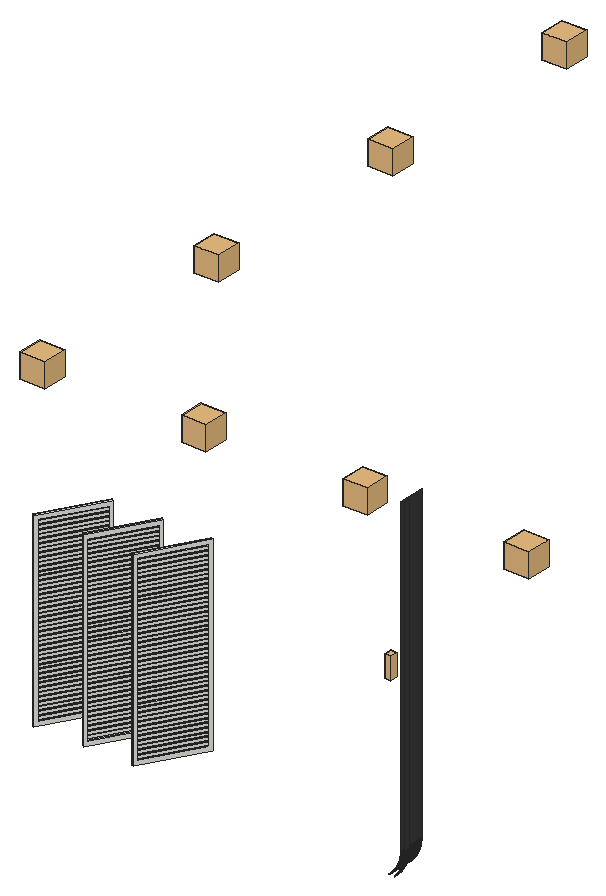
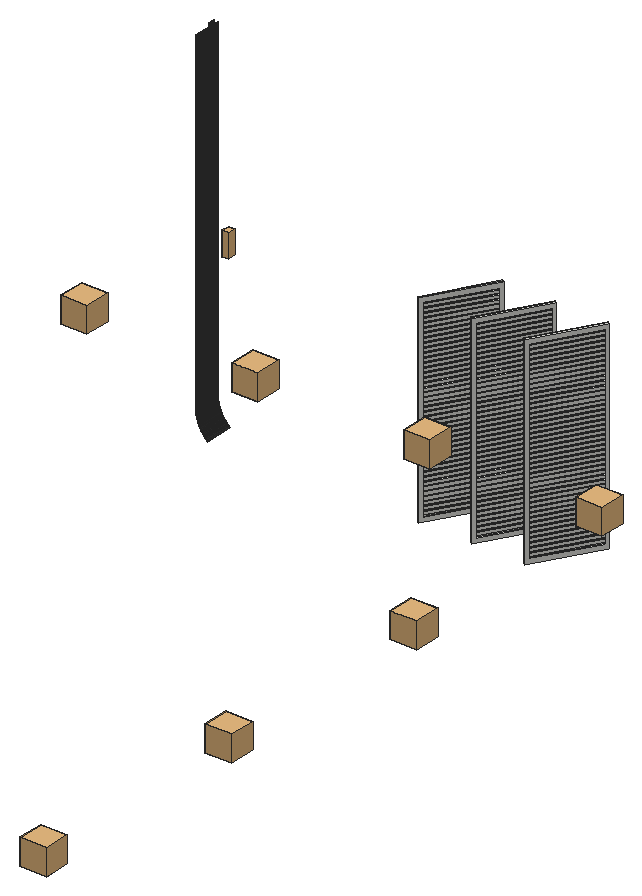
# SketchUp Ruby script. Lengths in inches.
U = 1.inch
M = Sketchup.active_model
def pt(a) = Geom::Point3d.new(a.map { |v| v * U })
def face(e, loops, mat)
  f = e.add_face(loops[0].map { |a| pt(a) })
  loops[1..].each { |l| e.add_face(l.map { |a| pt(a) }).erase! }
  f.material = f.back_material = mat if mat
  f
end
# faces: each face lists its corners as indices into pts; further lists are holes
def faces(e, pts, list, mat = nil) = list.each { |f| face(e, (f[0].is_a?(Array) ? f : [f]).map { |l| l.map { |i| pts[i] } }, mat) }
# xy, xz, yz: faces in a plane at the given z, y or x. An outline is a flat list of corners, or four numbers for a rectangle; further outlines are holes
def ring(l) = l.size == 4 ? [[l[0], l[1]], [l[2], l[1]], [l[2], l[3]], [l[0], l[3]]] : l.each_slice(2).to_a
def flat(e, list, mat, &to3) = list.each { |f| face(e, (f[0].is_a?(Array) ? f : [f]).map { |l| ring(l).map { |u, v| to3.(u, v) } }, mat) }
def xy(e, z, list, mat = nil) = flat(e, list, mat) { |x, y| [x, y, z] }
def xz(e, y, list, mat = nil) = flat(e, list, mat) { |x, z| [x, y, z] }
def yz(e, x, list, mat = nil) = flat(e, list, mat) { |y, z| [x, y, z] }
def lines(e, pts, list) = list.each { |a, b| e.add_line(pt(pts[a]), pt(pts[b])) }
# prism: a flat outline (further loops are holes) pulled along v
def prism(e, loops, v, mat = nil)
  f = face(e, loops, mat); d = Geom::Vector3d.new(v.map { |x| x * U })
  f.pushpull(f.normal.samedirection?(d) ? d.length : -d.length)
end
def box(e, o, s, mat = nil) = prism(e, [[o, [o[0] + s[0], o[1], o[2]], [o[0] + s[0], o[1] + s[1], o[2]], [o[0], o[1] + s[1], o[2]]]], [0, 0, s[2]], mat)
def at(x, y, z, deg = 0) = Geom::Transformation.translation(pt([x, y, z])) * Geom::Transformation.rotation(ORIGIN, Z_AXIS, deg.degrees)
def axes(o, x, y, z) = Geom::Transformation.new([*x, 0, *y, 0, *z, 0, *pt(o).to_a, 1])
def part(name) = M.definitions.add(name)
# library, detail: a bought-in or finely detailed component or shape, given as its bounding box
def library(name, o, s) = part(name).tap { |d| box(d.entities, o, s) }
def detail(e, o, s) = box(e.add_group.entities, o, s)
def put(e, d, t, mat = nil) = e.add_instance(d, t).tap { |i| i.material = mat if mat }
def group(e, t, mat = nil) = e.add_group.tap { |g| g.transformation = t; g.material = mat if mat }.entities
root = M.entities
M.materials.add("1496 AP 8293 CARBON COPY").color = [58, 58, 58]
c1 = part("1")
box(c1.entities,[-0.25,-0.25,0],[1,1,33])
c2 = part("Group\#27")
prism(c2.entities,[[[36,0,0],[0,0,0],[0,0,72],[36,0,72]],[[34.5,0,1.5],[34.5,0,70.5],[1.5,0,70.5],[1.5,0,1.5]]],[0,-1.5,0])
put(c2.entities,c1,axes([1.5,-1,2.5],[0,1,0],[0,0,1],[1,0,0]))
put(c2.entities,c1,axes([1.5,-1,4.08],[0,1,0],[0,0,1],[1,0,0]))
put(c2.entities,c1,axes([1.5,-1,5.67],[0,1,0],[0,0,1],[1,0,0]))
put(c2.entities,c1,axes([1.5,-1,7.25],[0,1,0],[0,0,1],[1,0,0]))
put(c2.entities,c1,axes([1.5,-1,8.83],[0,1,0],[0,0,1],[1,0,0]))
put(c2.entities,c1,axes([1.5,-1,10.42],[0,1,0],[0,0,1],[1,0,0]))
put(c2.entities,c1,axes([1.5,-1,12],[0,1,0],[0,0,1],[1,0,0]))
put(c2.entities,c1,axes([1.5,-1,13.58],[0,1,0],[0,0,1],[1,0,0]))
put(c2.entities,c1,axes([1.5,-1,15.17],[0,1,0],[0,0,1],[1,0,0]))
put(c2.entities,c1,axes([1.5,-1,16.75],[0,1,0],[0,0,1],[1,0,0]))
put(c2.entities,c1,axes([1.5,-1,18.33],[0,1,0],[0,0,1],[1,0,0]))
put(c2.entities,c1,axes([1.5,-1,19.92],[0,1,0],[0,0,1],[1,0,0]))
put(c2.entities,c1,axes([1.5,-1,21.5],[0,1,0],[0,0,1],[1,0,0]))
put(c2.entities,c1,axes([1.5,-1,23.08],[0,1,0],[0,0,1],[1,0,0]))
put(c2.entities,c1,axes([1.5,-1,24.67],[0,1,0],[0,0,1],[1,0,0]))
put(c2.entities,c1,axes([1.5,-1,26.25],[0,1,0],[0,0,1],[1,0,0]))
put(c2.entities,c1,axes([1.5,-1,27.83],[0,1,0],[0,0,1],[1,0,0]))
put(c2.entities,c1,axes([1.5,-1,29.42],[0,1,0],[0,0,1],[1,0,0]))
put(c2.entities,c1,axes([1.5,-1,31],[0,1,0],[0,0,1],[1,0,0]))
put(c2.entities,c1,axes([1.5,-1,32.58],[0,1,0],[0,0,1],[1,0,0]))
put(c2.entities,c1,axes([1.5,-1,34.17],[0,1,0],[0,0,1],[1,0,0]))
put(c2.entities,c1,axes([1.5,-1,35.75],[0,1,0],[0,0,1],[1,0,0]))
put(c2.entities,c1,axes([1.5,-1,37.33],[0,1,0],[0,0,1],[1,0,0]))
put(c2.entities,c1,axes([1.5,-1,38.92],[0,1,0],[0,0,1],[1,0,0]))
put(c2.entities,c1,axes([1.5,-1,40.5],[0,1,0],[0,0,1],[1,0,0]))
put(c2.entities,c1,axes([1.5,-1,42.08],[0,1,0],[0,0,1],[1,0,0]))
put(c2.entities,c1,axes([1.5,-1,43.67],[0,1,0],[0,0,1],[1,0,0]))
put(c2.entities,c1,axes([1.5,-1,45.25],[0,1,0],[0,0,1],[1,0,0]))
put(c2.entities,c1,axes([1.5,-1,46.83],[0,1,0],[0,0,1],[1,0,0]))
put(c2.entities,c1,axes([1.5,-1,48.42],[0,1,0],[0,0,1],[1,0,0]))
put(c2.entities,c1,axes([1.5,-1,50],[0,1,0],[0,0,1],[1,0,0]))
put(c2.entities,c1,axes([1.5,-1,51.58],[0,1,0],[0,0,1],[1,0,0]))
put(c2.entities,c1,axes([1.5,-1,53.17],[0,1,0],[0,0,1],[1,0,0]))
put(c2.entities,c1,axes([1.5,-1,54.75],[0,1,0],[0,0,1],[1,0,0]))
put(c2.entities,c1,axes([1.5,-1,56.33],[0,1,0],[0,0,1],[1,0,0]))
put(c2.entities,c1,axes([1.5,-1,57.92],[0,1,0],[0,0,1],[1,0,0]))
put(c2.entities,c1,axes([1.5,-1,59.5],[0,1,0],[0,0,1],[1,0,0]))
put(c2.entities,c1,axes([1.5,-1,61.08],[0,1,0],[0,0,1],[1,0,0]))
put(c2.entities,c1,axes([1.5,-1,62.67],[0,1,0],[0,0,1],[1,0,0]))
put(c2.entities,c1,axes([1.5,-1,64.25],[0,1,0],[0,0,1],[1,0,0]))
put(c2.entities,c1,axes([1.5,-1,65.83],[0,1,0],[0,0,1],[1,0,0]))
put(c2.entities,c1,axes([1.5,-1,67.42],[0,1,0],[0,0,1],[1,0,0]))
put(c2.entities,c1,axes([1.5,-1,69],[0,1,0],[0,0,1],[1,0,0]))
c3 = library("WALL LIGHT 69",[4.19,4.05,-8.78],[4.61,5.7,17.13])
c4 = library("2",[-4.69,-4.69,-13.16],[13.38,13.38,13.16])
yz(root,308.99,[[71,160.29,85,160.53]],"1496 AP 8293 CARBON COPY")
yz(root,309,[[71,160.76,85,161],[71,161,85,331]],"1496 AP 8293 CARBON COPY")
yz(root,311,[[71,160.74,74,161],[71,161,74,331]],"1496 AP 8293 CARBON COPY")
p = [[305.6875,71,147.42],[305.51,71,147.23],[305.51,74,147.23],[305.6875,74,147.42],[302.69,71,147.3125],[302.87,71,147.47],
  [302.87,85,147.47],[302.69,85,147.3125],[305.86,71,147.62],[305.86,74,147.62],[303.04,71,147.625],[303.04,85,147.625],
  [303.22,71,147.78],[303.22,85,147.78],[306.04,71,147.8125],[306.04,74,147.8125],[303.39,71,147.94],[303.39,85,147.94],
  [306.21,71,148.01],[306.21,74,148.01],[303.56,71,148.11],[303.56,85,148.11],[306.375,71,148.21],[306.375,74,148.21],
  [303.73,71,148.27],[303.73,85,148.27],[306.54,71,148.41],[306.54,74,148.41],[303.89,71,148.44],[303.89,85,148.44],
  [304.06,71,148.61],[304.06,85,148.61],[306.71,71,148.62],[306.71,74,148.62],[304.22,71,148.78],[304.22,85,148.78],
  [306.87,71,148.82],[306.87,74,148.82],[304.375,71,148.96],[304.375,85,148.96],[307.03,71,149.03],[307.03,74,149.03],
  [304.53,71,149.13],[304.53,85,149.13],[307.18,71,149.24],[307.18,74,149.24],[304.6875,71,149.31],[304.6875,85,149.31],
  [307.33,71,149.46],[307.33,74,149.46],[304.84,71,149.49],[304.84,85,149.49],[304.99,71,149.67],[304.99,85,149.67],
  [307.48,71,149.67],[307.48,74,149.67],[305.14,71,149.86],[305.14,85,149.86],[307.63,71,149.89],[307.63,74,149.89],
  [305.28,71,150.04],[305.28,85,150.04],[307.77,71,150.11],[307.77,74,150.11],[305.42,71,150.23],[305.42,85,150.23],
  [307.91,71,150.33],[307.91,74,150.33],[305.5625,71,150.42],[305.5625,85,150.42],[308.05,71,150.55],[308.05,74,150.55],
  [305.7,71,150.61],[305.7,85,150.61],[305.83,71,150.8],[305.83,85,150.8],[308.1875,71,150.77],[308.1875,74,150.77],
  [305.97,71,151],[305.97,85,151],[308.32,71,151],[308.32,74,151],[306.1,71,151.2],[306.1,85,151.2],
  [308.45,71,151.23],[308.45,74,151.23],[306.22,71,151.39],[306.22,85,151.39],[308.58,71,151.46],[308.58,74,151.46],
  [306.35,71,151.6],[306.35,85,151.6],[308.7,71,151.6875],[308.7,74,151.6875],[306.47,71,151.8],[306.47,85,151.8],
  [308.82,71,151.92],[308.82,74,151.92],[306.59,71,152],[306.59,85,152],[308.9375,71,152.15],[308.9375,74,152.15],
  [306.7,71,152.2],[306.7,85,152.2],[306.82,71,152.41],[306.82,85,152.41],[309.05,71,152.39],[309.05,74,152.39],
  [306.93,71,152.62],[306.93,85,152.62],[309.16,71,152.625],[309.16,74,152.625],[307.04,71,152.83],[307.04,85,152.83],
  [309.27,71,152.87],[309.27,74,152.87],[307.14,71,153.04],[307.14,85,153.04],[309.375,71,153.11],[309.375,74,153.11],
  [307.25,71,153.25],[307.25,85,153.25],[309.48,71,153.35],[309.48,74,153.35],[307.35,71,153.46],[307.35,85,153.46],
  [309.58,71,153.59],[309.58,74,153.59],[307.44,71,153.68],[307.44,85,153.68],[309.67,71,153.83],[309.67,74,153.83],
  [307.54,71,153.89],[307.54,85,153.89],[309.76,71,154.08],[309.76,74,154.08],[307.63,71,154.11],[307.63,85,154.11],
  [307.72,71,154.33],[307.72,85,154.33],[309.85,71,154.32],[309.85,74,154.32],[307.8,71,154.55],[307.8,85,154.55],
  [309.9375,71,154.57],[309.9375,74,154.57],[307.89,71,154.77],[307.89,85,154.77],[310.02,71,154.82],[310.02,74,154.82],
  [307.97,71,154.99],[307.97,85,154.99],[310.1,71,155.07],[310.1,74,155.07],[308.04,71,155.21],[308.04,85,155.21],
  [310.18,71,155.32],[310.18,74,155.32],[308.12,71,155.4375],[308.12,85,155.4375],[310.25,71,155.57],[310.25,74,155.57],
  [308.19,71,155.66],[308.19,85,155.66],[310.32,71,155.82],[310.32,74,155.82],[308.26,71,155.89],[308.26,85,155.89],
  [310.38,71,156.08],[310.38,74,156.08],[308.32,71,156.11],[308.32,85,156.11],[308.39,71,156.34],[308.39,85,156.34],
  [310.45,71,156.33],[310.45,74,156.33],[308.45,71,156.57],[308.45,85,156.57],[310.51,71,156.59],[310.51,74,156.59],
  [308.5,71,156.8],[308.5,85,156.8],[310.5625,71,156.84],[310.5625,74,156.84],[308.56,71,157.03],[308.56,85,157.03],
  [310.62,71,157.1],[310.62,74,157.1],[308.61,71,157.26],[308.61,85,157.26],[310.67,71,157.36],[310.67,74,157.36],
  [308.65,71,157.49],[308.65,85,157.49],[310.71,71,157.61],[310.71,74,157.61],[308.7,71,157.72],[308.7,85,157.72],
  [310.75,71,157.87],[310.75,74,157.87],[308.74,71,157.95],[308.74,85,157.95],[310.79,71,158.13],[310.79,74,158.13],
  [308.78,71,158.18],[308.78,85,158.18],[310.83,71,158.39],[310.83,74,158.39],[308.8125,71,158.42],[308.8125,85,158.42],
  [308.85,71,158.65],[308.85,85,158.65],[310.86,71,158.65],[310.86,74,158.65],[310.89,71,158.91],[310.89,74,158.91],
  [308.875,71,158.88],[308.875,85,158.88],[308.9,71,159.12],[308.9,85,159.12],[310.92,71,159.17],[310.92,74,159.17],
  [308.92,71,159.35],[308.92,85,159.35],[310.9375,71,159.43],[310.9375,74,159.43],[308.94,71,159.59],[308.94,85,159.59],
  [310.96,71,159.69],[310.96,74,159.69],[308.96,71,159.82],[308.96,85,159.82],[310.97,71,159.95],[310.97,74,159.95],
  [308.98,71,160.06],[308.98,85,160.06],[310.98,71,160.21],[310.98,74,160.21],[308.99,71,160.29],[308.99,85,160.29],
  [310.99,71,160.48],[310.99,74,160.48],[308.99,71,160.53],[309,71,160.76],[309,85,160.76],[308.99,85,160.53],
  [311,71,160.74],[311,74,160.74]]
faces(root,p,[[0,1,2,3],[4,5,6,7],[8,0,3,9],[5,10,11,6],[10,12,13,11],[14,8,9,15],[12,16,17,13],[18,14,15,19],
  [16,20,21,17],[22,18,19,23],[20,24,25,21],[26,22,23,27],[24,28,29,25],[28,30,31,29],[32,26,27,33],[30,34,35,31],
  [36,32,33,37],[34,38,39,35],[40,36,37,41],[38,42,43,39],[44,40,41,45],[42,46,47,43],[48,44,45,49],[46,50,51,47],
  [50,52,53,51],[54,48,49,55],[52,56,57,53],[58,54,55,59],[56,60,61,57],[62,58,59,63],[60,64,65,61],[66,62,63,67],
  [64,68,69,65],[70,66,67,71],[68,72,73,69],[72,74,75,73],[76,70,71,77],[74,78,79,75],[80,76,77,81],[78,82,83,79],
  [84,80,81,85],[82,86,87,83],[88,84,85,89],[86,90,91,87],[92,88,89,93],[90,94,95,91],[96,92,93,97],[94,98,99,95],
  [100,96,97,101],[98,102,103,99],[102,104,105,103],[106,100,101,107],[104,108,109,105],[110,106,107,111],[108,112,113,109],[114,110,111,115],
  [112,116,117,113],[118,114,115,119],[116,120,121,117],[122,118,119,123],[120,124,125,121],[126,122,123,127],[124,128,129,125],[130,126,127,131],
  [128,132,133,129],[134,130,131,135],[132,136,137,133],[136,138,139,137],[140,134,135,141],[138,142,143,139],[144,140,141,145],[142,146,147,143],
  [148,144,145,149],[146,150,151,147],[152,148,149,153],[150,154,155,151],[156,152,153,157],[154,158,159,155],[160,156,157,161],[158,162,163,159],
  [164,160,161,165],[162,166,167,163],[168,164,165,169],[166,170,171,167],[170,172,173,171],[174,168,169,175],[172,176,177,173],[178,174,175,179],
  [176,180,181,177],[182,178,179,183],[180,184,185,181],[186,182,183,187],[184,188,189,185],[190,186,187,191],[188,192,193,189],[194,190,191,195],
  [192,196,197,193],[198,194,195,199],[196,200,201,197],[202,198,199,203],[200,204,205,201],[206,202,203,207],[204,208,209,205],[208,210,211,209],
  [212,206,207,213],[214,212,213,215],[210,216,217,211],[216,218,219,217],[220,214,215,221],[218,222,223,219],[224,220,221,225],[222,226,227,223],
  [228,224,225,229],[226,230,231,227],[232,228,229,233],[230,234,235,231],[236,232,233,237],[234,238,239,235],[240,236,237,241],[242,243,244,245],
  [246,240,241,247]],"1496 AP 8293 CARBON COPY")
put(root,c2,axes([113.76,65.07,155.97],[0.5,0.86603,0],[-0.86603,0.5,0],[0,0,1.43056]))
put(root,c2,axes([140.76,65.07,155.97],[0.5,0.86603,0],[-0.86603,0.5,0],[0,0,1.43056]))
put(root,c2,axes([167.76,65.07,155.97],[0.5,0.86603,0],[-0.86603,0.5,0],[0,0,1.43056]))
put(root,c3,axes([289.27,78.18,240.75],[0.7,0,0],[0,0.7,0],[0,0,0.7]))
put(root,c4,at(27,175.5,259.2))
put(root,c4,at(27,293.67,259.2))
put(root,c4,at(27,411.83,259.2))
put(root,c4,at(27,530,259.2))
put(root,c4,at(114.67,175.5,259.2))
put(root,c4,at(202.33,175.5,259.2))
put(root,c4,at(290,175.5,259.2))
